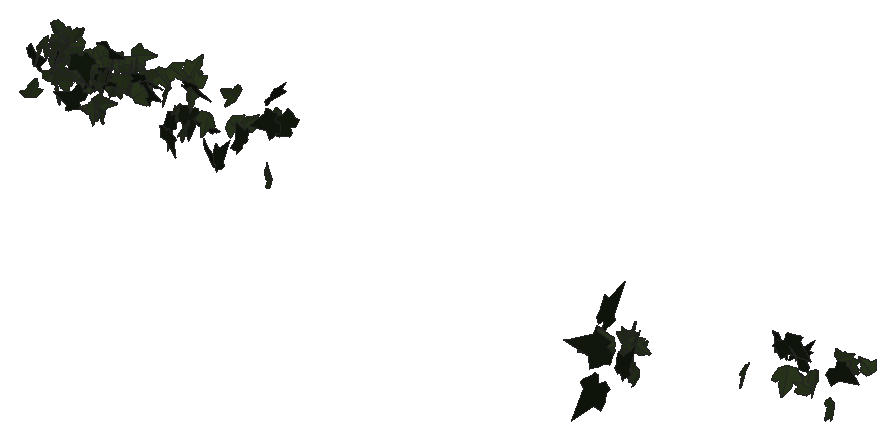
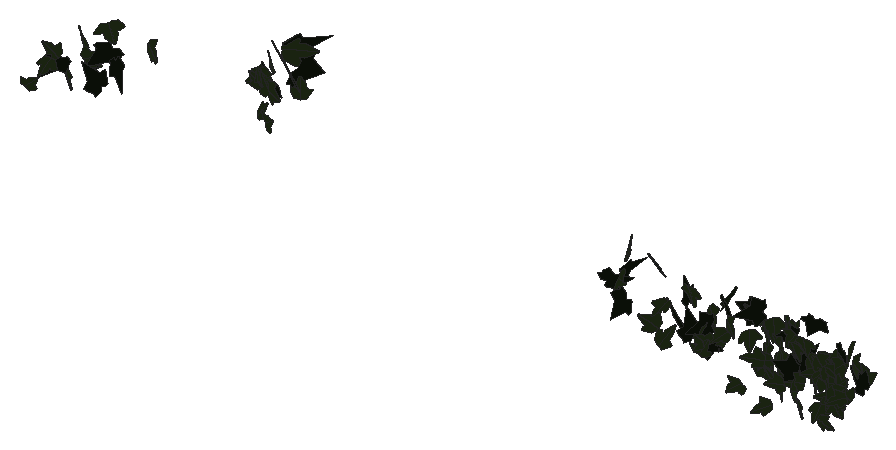
# SketchUp Ruby script. Lengths in inches.
U = 1.inch
M = Sketchup.active_model
def pt(a) = Geom::Point3d.new(a.map { |v| v * U })
def face(e, loops, mat)
  f = e.add_face(loops[0].map { |a| pt(a) })
  loops[1..].each { |l| e.add_face(l.map { |a| pt(a) }).erase! }
  f.material = f.back_material = mat if mat
  f
end
# faces: each face lists its corners as indices into pts; further lists are holes
def faces(e, pts, list, mat = nil) = list.each { |f| face(e, (f[0].is_a?(Array) ? f : [f]).map { |l| l.map { |i| pts[i] } }, mat) }
# xy, xz, yz: faces in a plane at the given z, y or x. An outline is a flat list of corners, or four numbers for a rectangle; further outlines are holes
def ring(l) = l.size == 4 ? [[l[0], l[1]], [l[2], l[1]], [l[2], l[3]], [l[0], l[3]]] : l.each_slice(2).to_a
def flat(e, list, mat, &to3) = list.each { |f| face(e, (f[0].is_a?(Array) ? f : [f]).map { |l| ring(l).map { |u, v| to3.(u, v) } }, mat) }
def xy(e, z, list, mat = nil) = flat(e, list, mat) { |x, y| [x, y, z] }
def xz(e, y, list, mat = nil) = flat(e, list, mat) { |x, z| [x, y, z] }
def yz(e, x, list, mat = nil) = flat(e, list, mat) { |y, z| [x, y, z] }
def lines(e, pts, list) = list.each { |a, b| e.add_line(pt(pts[a]), pt(pts[b])) }
# prism: a flat outline (further loops are holes) pulled along v
def prism(e, loops, v, mat = nil)
  f = face(e, loops, mat); d = Geom::Vector3d.new(v.map { |x| x * U })
  f.pushpull(f.normal.samedirection?(d) ? d.length : -d.length)
end
def box(e, o, s, mat = nil) = prism(e, [[o, [o[0] + s[0], o[1], o[2]], [o[0] + s[0], o[1] + s[1], o[2]], [o[0], o[1] + s[1], o[2]]]], [0, 0, s[2]], mat)
def at(x, y, z, deg = 0) = Geom::Transformation.translation(pt([x, y, z])) * Geom::Transformation.rotation(ORIGIN, Z_AXIS, deg.degrees)
def axes(o, x, y, z) = Geom::Transformation.new([*x, 0, *y, 0, *z, 0, *pt(o).to_a, 1])
def part(name) = M.definitions.add(name)
# library, detail: a bought-in or finely detailed component or shape, given as its bounding box
def library(name, o, s) = part(name).tap { |d| box(d.entities, o, s) }
def detail(e, o, s) = box(e.add_group.entities, o, s)
def put(e, d, t, mat = nil) = e.add_instance(d, t).tap { |i| i.material = mat if mat }
def group(e, t, mat = nil) = e.add_group.tap { |g| g.transformation = t; g.material = mat if mat }.entities
root = M.entities
M.materials.add("efeu1").color = [18, 25, 13]
M.materials.add("efeu2").color = [43, 57, 29]
c1 = part("ivyleaf_10")
p = [[0,0.5,-0.03],[-0.0625,2.02,-0.43],[-0.19,2.01,-0.46],[-0.54,1.05,-0.29],[-0.52,0.625,-0.18],[-0.83,0.76,-0.28],
  [-1.16,0.64,-0.33],[-1.15,0.33,-0.24],[-0.77,-0.39,0.02],[-0.3,-0.51,0.16],[0.04,-0.48,0.23],[-0.02,2.01,-0.4375],
  [-0.06,2.01,-0.43],[0.04,-0.49,0.23],[0.67,-0.49,0.14],[1.38,0.36,-0.2],[1.375,0.51,-0.24],[0.81,0.65,-0.19],
  [0.62,0.59,-0.15],[0.6,1.09,-0.28],[0.5,1.23,-0.31]]
faces(c1.entities,p,[[0,1,2,3,4,5,6,7,8,9,10],[11,12,0,13,14,15,16,17,18,19,20]],"efeu2")
c2 = part("ivyleaf_9")
p = [[1.54,2.16,1.25],[1.36,2.04,1.19],[-0.21,0.99,0.68],[-0.71,1.11,0.82],[-0.85,0.86,0.67],[-0.8,0.17,0.21],
  [-0.9,-0.01,0.1],[-0.67,-0.16,-0.02],[-0.08,-0.08,-0.05],[-0.03,-0.6,-0.4],[0.65,-0.88,-0.66],[0.83,-0.6,-0.49],
  [1.29,-0.42,-0.43],[1.8125,-0.07,-0.26],[1.21,0.44,0.15]]
faces(c2.entities,p,[[0,1,2,3,4,5,6,7,8,9,10,11,12,13,14]],"efeu1")
put(root,c1,axes([519.28,138.82,150.8125],[0.15323,0.09847,0.63212],[0.38291,0.50659,-0.17174],[-0.51249,0.40794,0.06068]))
put(root,c1,axes([519.85,138.97,149.92],[0.47339,0.37363,-0.23743],[-0.18464,-0.14928,-0.60307],[-0.40234,0.50812,-0.00259]))
put(root,c2,axes([519.46,135.91,150.5],[0.0764,-0.09138,0.78277],[0.4972,-0.60459,-0.11911],[0.61145,0.50304,-0.00095]))
put(root,c1,axes([520.43,139.92,148.9],[0.20455,-0.06424,-0.6006],[-0.57771,0.16432,-0.21433],[0.17635,0.61283,-0.00548]))
put(root,c1,axes([520.34,138.58,151.12],[-0.29048,-0.52947,0.26685],[-0.12391,-0.23638,-0.6039],[0.57982,-0.31577,0.00463]))
put(root,c1,axes([520.6,136.84,150.53],[-0.11991,0.37286,0.53038],[-0.20002,0.49179,-0.39096],[-0.6167,-0.232,0.02367]))
put(root,c1,axes([520.39,135.74,152.08],[0.31226,-0.53217,0.51218],[0.25786,-0.44253,-0.61701],[0.69212,0.40496,-0.0012]))
put(root,c1,axes([520.28,137.75,153.01],[-0.52251,0.1784,-0.50215],[0.47077,-0.17499,-0.55204],[-0.2497,-0.70324,0.00998]))
put(root,c1,axes([520.93,137.53,151.31],[-0.24196,-0.66163,0.09856],[-0.03519,-0.09208,-0.70448],[0.66801,-0.2445,-0.00141]))
put(root,c1,axes([520.78,136.25,149.17],[-0.26522,-0.44928,0.37864],[0.18614,0.32978,0.52169],[-0.55729,0.32397,-0.00596]))
put(root,c1,axes([521.37,138.68,149.34],[-0.16271,0.16443,-0.63572],[-0.4383,0.4605,0.23129],[0.48895,0.46751,-0.00423]))
put(root,c1,axes([520.69,137.91,150.44],[0.27064,-0.32237,0.5824],[0.40891,-0.41558,-0.42005],[0.52526,0.48963,0.02692]))
put(root,c1,axes([521.08,139.42,149.67],[-0.46445,-0.38016,-0.22724],[0.1756,0.14424,-0.6002],[0.4066,-0.49653,-0.00037]))
put(root,c1,axes([521.21,137.8,151.26],[0.05305,-0.69928,-0.18249],[-0.01026,0.18224,-0.70128],[0.72263,0.05392,0.00344]))
put(root,c1,axes([521.31,138.21,152.42],[-0.21036,-0.48272,0.36837],[-0.12313,-0.34784,-0.52613],[0.5946,-0.24281,0.02137]))
put(root,c1,axes([521.47,136.4,149.61],[0.43935,-0.46341,-0.33146],[-0.23385,0.23501,-0.63854],[0.51955,0.49766,-0.00712]))
put(root,c1,axes([520.83,138.28,152.01],[0.12747,-0.08265,-0.6202],[0.60457,-0.14678,0.14381],[-0.16118,-0.61592,0.04895]))
put(root,c1,axes([521.54,134.72,152.92],[-0.35621,0.53889,0.4395],[-0.2419,0.36694,-0.64598],[-0.65196,-0.43058,-0.00045]))
put(root,c1,axes([521.27,136.45,151.65],[-0.57958,0.12039,0.3449],[0.3385,-0.06626,0.59194],[0.13738,0.67118,-0.00343]))
put(root,c1,axes([521.39,133.22,149.22],[-0.38018,-0.60564,0.09897],[0.05569,0.08189,0.71507],[-0.61114,0.38422,0.0036]))
put(root,c1,axes([522,137.86,151.08],[-0.11217,-0.53913,0.45324],[-0.12197,-0.43715,-0.55018],[0.6937,-0.16404,-0.02345]))
put(root,c1,axes([522.21,138.11,152.95],[-0.07747,-0.65397,0.2853],[-0.05103,-0.28116,-0.65834],[0.71167,-0.09135,-0.01615]))
put(root,c1,axes([522.25,138.33,151.43],[-0.01249,0.25001,0.63304],[0.03478,-0.63209,0.25032],[0.67973,0.03694,-0.00118]))
put(root,c1,axes([521.82,137.05,149.24],[0.03179,-0.06086,0.66522],[0.52325,0.41626,0.01307],[-0.41525,0.51986,0.06741]))
put(root,c2,axes([522.76,134.5,151.98],[-0.29334,0.20895,-0.70547],[-0.61317,0.35034,0.35873],[0.40666,0.67897,0.032]))
put(root,c1,axes([522.72,134.96,148.48],[-0.16462,0.31635,-0.57425],[-0.27755,0.50277,0.35654],[0.59397,0.32262,0.00745]))
put(root,c1,axes([523.15,134.54,151.41],[-0.08346,-0.55043,-0.56858],[0.12144,0.55605,-0.55613],[0.78199,-0.1451,0.02568]))
put(root,c1,axes([523.82,135.9,151.52],[0.10232,0.00181,-0.71091],[-0.66095,0.26474,-0.09446],[0.2618,0.66766,0.03938]))
put(root,c1,axes([523.25,136.72,150.7],[-0.06403,-0.11847,0.71745],[0.3516,0.62539,0.13465],[-0.63651,0.35737,0.0022]))
put(root,c1,axes([523.77,138.77,148.93],[0.48635,-0.44559,-0.15978],[-0.11213,0.11412,-0.65956],[0.4599,0.49904,0.00816]))
put(root,c1,axes([523.25,134.55,150.44],[-0.3655,-0.1091,0.69788],[0.69173,0.10379,0.37851],[-0.143,0.78093,0.04719]))
put(root,c1,axes([524.48,135.93,149.6],[0.34307,-0.54592,-0.33052],[-0.18009,0.27718,-0.64476],[0.61224,0.38744,-0.00444]))
put(root,c2,axes([524.76,134.91,149],[-0.0473,-0.01374,0.76617],[-0.71265,-0.28136,-0.04904],[0.28166,-0.7142,0.00458]))
put(root,c1,axes([524.8,135.92,151.05],[0.08578,-0.7222,0.17778],[0.01533,-0.1772,-0.72725],[0.7436,0.08696,-0.00551]))
put(root,c1,axes([524.49,138.49,149.54],[0.23113,-0.26019,0.60981],[0.38881,-0.4699,-0.34786],[0.53702,0.45219,-0.0106]))
put(root,c2,axes([524.25,138.86,151.52],[0.31958,-0.15421,0.67829],[0.58557,-0.34327,-0.35394],[0.37546,0.66662,-0.02534]))
put(root,c1,axes([525.07,136.21,152.76],[0.69435,0.04049,0.03455],[0.0345,0.0019,-0.69553],[-0.04054,0.6952,-0.00011]))
put(root,c1,axes([524.78,135.41,150.41],[0.42243,-0.04589,-0.61922],[0.62048,0.00287,0.42308],[-0.02349,-0.74959,0.03953]))
put(root,c2,axes([525.51,136.22,150.41],[0.14984,0.1017,0.75128],[-0.61338,-0.43382,0.18106],[0.44557,-0.63141,-0.00339]))
put(root,c1,axes([525.39,137.1875,152.69],[0.66964,-0.14152,-0.14354],[-0.14068,0.02853,-0.68443],[0.14436,0.68426,-0.00115]))
put(root,c1,axes([524.82,139.68,150.57],[0.15558,0.07308,0.70938],[0.66733,0.2411,-0.17119],[-0.25146,0.68505,-0.01543]))
put(root,c1,axes([525.99,138.32,149.67],[0.30028,-0.55214,-0.34084],[-0.16407,0.29875,-0.62851],[0.62779,0.34218,-0.00123]))
put(root,c1,axes([525.84,135.34,151.9],[-0.32458,-0.31187,-0.51603],[0.38467,0.34418,-0.44997],[0.46431,-0.50317,0.01205]))
put(root,c2,axes([525.76,134.1,153.55],[-0.36013,-0.38511,-0.59413],[0.4411,0.39938,-0.52625],[0.55384,-0.5685,0.03278]))
put(root,c1,axes([525.85,140.02,148.4],[0.12134,0.12235,0.65875],[0.2887,0.59458,-0.16361],[-0.60462,0.30846,0.05408]))
put(root,c1,axes([525.77,139.21,150.63],[0.13979,-0.09929,-0.65288],[0.56403,-0.32916,0.17083],[-0.34349,-0.5809,0.0148]))
put(root,c1,axes([525.87,135.9375,148.68],[0.01511,-0.0893,0.72977],[0.46504,0.56652,0.05969],[-0.56945,0.46027,0.06811]))
put(root,c1,axes([526.26,136.93,150.2],[-0.02624,0.29922,0.63077],[-0.01742,0.63073,-0.29993],[-0.69792,-0.02699,-0.01623]))
put(root,c1,axes([526.56,135.83,148.89],[0.0242,0.02446,-0.67286],[-0.3282,-0.58746,-0.03316],[-0.58789,0.32897,-0.00919]))
put(root,c1,axes([527.09,134.13,149.08],[-0.00863,0.02124,0.74142],[-0.72904,-0.13679,-0.00457],[0.1366,-0.72875,0.02247]))
put(root,c1,axes([526.09,135.29,151.45],[0.00567,0.00174,-0.68587],[0.57809,-0.36912,0.00385],[-0.36909,-0.5781,-0.00452]))
put(root,c1,axes([526.45,135.86,152.6],[0.62395,0.13375,0.4526],[0.44342,0.09078,-0.63811],[-0.16161,0.76545,-0.00341]))
put(root,c1,axes([527.62,136.16,150.59],[-0.51443,0.03771,0.49433],[-0.49479,0.00559,-0.51534],[-0.03106,-0.71342,0.02209]))
put(root,c1,axes([527.4,136.375,150.7],[0.06144,-0.60006,-0.46953],[-0.06153,0.46561,-0.6031],[0.75943,0.08627,-0.01088]))
put(root,c1,axes([526.92,138.55,151.48],[-0.10123,-0.04001,-0.67305],[0.67346,0.02672,-0.10288],[0.03241,-0.6801,0.03555]))
put(root,c1,axes([527.71,133.9,152.02],[-0.15439,0.152,0.68158],[-0.44258,0.51865,-0.21592],[-0.54017,-0.46839,-0.0179]))
put(root,c1,axes([527.57,134.92,152.71],[0.28299,-0.73749,-0.12828],[-0.04111,0.12162,-0.7899],[0.74743,0.28591,0.00512]))
put(root,c1,axes([527.03,139.5,151.91],[-0.08148,-0.04365,0.74271],[0.56265,0.48522,0.09024],[-0.48677,0.56817,-0.02]))
put(root,c1,axes([527.7,137.99,149.67],[0.54286,0.39171,0.27104],[-0.22529,-0.15094,0.66937],[0.41969,-0.58769,0.00873]))
put(root,c2,axes([526.95,134.99,152.09],[0.19712,0.03102,-0.74405],[0.59548,0.45561,0.17676],[0.44718,-0.62039,0.0926]))
put(root,c1,axes([527.23,133.67,150.02],[0.57991,-0.24788,0.42428],[0.39044,-0.16605,-0.63066],[0.29836,0.6991,0.00064]))
put(root,c1,axes([527.8,138.32,151.58],[0.10849,-0.37254,-0.59541],[-0.1209,0.58357,-0.38716],[0.69187,0.16039,0.0257]))
put(root,c1,axes([528.13,134.73,152.9375],[0.25513,-0.60969,-0.39956],[-0.14373,0.37294,-0.66085],[0.71464,0.29267,0.00973]))
put(root,c1,axes([528.18,135.6,151.11],[0.55412,-0.1744,0.3643],[-0.3468,0.11159,0.58091],[-0.20704,-0.65369,0.00197]))
put(root,c1,axes([527.8125,133.83,149.43],[-0.39522,0.09706,0.58681],[0.55217,-0.20199,0.4053],[0.22107,0.67804,0.03674]))
put(root,c1,axes([528.46,136.875,151.34],[0.19846,-0.71041,-0.10598],[-0.0173,0.10519,-0.73752],[0.71806,0.19888,0.01153]))
put(root,c1,axes([528.01,140.9,149.91],[0.42299,0.17543,0.57575],[0.53208,0.21996,-0.45792],[-0.28135,0.67972,-0.00041]))
put(root,c1,axes([528.93,136.14,151.74],[0.50196,-0.45893,0.37581],[-0.27847,0.25238,0.68013],[-0.52375,-0.57402,-0.00143]))
put(root,c1,axes([529.17,135.125,152.54],[-0.56595,-0.51041,0.04357],[-0.03167,-0.02994,-0.76211],[0.51129,-0.56683,0.00102]))
put(root,c1,axes([529.85,137.32,152.22],[-0.47161,-0.55993,0.02203],[-0.00338,-0.02595,-0.73194],[0.56035,-0.47141,0.01412]))
put(root,c2,axes([530.58,134.92,152.96],[0.61995,-0.01156,0.4639],[0.464,0.00372,-0.61998],[0.00702,0.77429,0.00991]))
put(root,c1,axes([531.07,134.43,151.96],[0.47579,0.00884,-0.63596],[0.63585,0.01184,0.47587],[0.01478,-0.79415,0.00002]))
put(root,c1,axes([531.23,138.71,152.42],[0.31623,0.28971,0.5744],[0.38094,0.43144,-0.42733],[-0.51841,0.49375,0.03637]))
put(root,c2,axes([531.49,134.72,152.5],[0.39737,-0.07569,-0.68942],[0.67536,0.22307,0.36477],[0.15786,-0.76383,0.17485]))
put(root,c1,axes([532.08,140.05,151.94],[0.30368,0.44876,-0.52822],[0.25876,0.46159,0.54092],[0.64299,-0.3977,0.03178]))
put(root,c1,axes([532.5,140.09,150.95],[0.64187,0.264,0.30917],[-0.28736,-0.11409,0.69403],[0.28758,-0.70325,0.00347]))
put(root,c1,axes([532.41,136.63,152.01],[0.31407,-0.64295,0.2168],[0.10808,-0.18844,-0.71542],[0.66985,0.33187,0.01379]))
put(root,c1,axes([533.39,136.11,149.96],[0.11314,-0.24235,0.70677],[-0.35097,0.61382,0.26666],[-0.65961,-0.36817,-0.02066]))
put(root,c2,axes([533.36,137.88,152.06],[0.6978,-0.08585,0.31372],[0.30974,-0.05121,-0.70296],[0.09925,0.76336,-0.01187]))
put(root,c1,axes([533.87,137.74,151.73],[-0.04627,0.70809,-0.26757],[0.01701,-0.26702,-0.7096],[-0.75677,-0.0493,0.00041]))
put(root,c2,axes([533.93,137.5,150.0625],[-0.45402,-0.49592,-0.38339],[0.26365,0.2784,-0.67234],[0.56869,-0.52499,0.00562]))
put(root,c2,axes([535.125,133.6875,151.57],[-0.54015,0.06198,-0.66742],[0.66553,-0.05239,-0.54348],[-0.07975,-0.85701,-0.01504]))
put(root,c1,axes([535.97,140.65,150.93],[-0.22632,-0.39702,-0.64952],[-0.32556,-0.56204,0.45699],[-0.68812,0.39649,-0.00258]))
put(root,c1,axes([536.05,134.3,150.88],[0.13656,-0.72766,-0.02306],[-0.00475,0.02257,-0.74036],[0.72801,0.13664,-0.0005]))
put(root,c2,axes([535.78,132.3,151.21],[0.36248,-0.66754,0.13765],[0.06189,-0.12302,-0.75959],[0.67877,0.3677,-0.00425]))
put(root,c2,axes([536,136.76,149.85],[0.77113,0.02402,-0.01539],[0.01467,0.02324,0.77117],[0.02447,-0.77093,0.02277]))
put(root,c1,axes([537.9375,134.6,152.25],[0.80025,-0.1316,-0.0261],[-0.02516,0.00785,-0.81099],[0.13178,0.80064,0.00366]))
put(root,c1,axes([538.76,138.125,150.25],[-0.31512,-0.40181,0.57351],[0.35372,0.45143,0.51064],[-0.60435,0.47373,-0.00017]))
put(root,c2,axes([539.05,134.49,148.66],[-0.32282,0.52243,0.57369],[0.30287,-0.48723,0.61412],[0.71437,0.44266,-0.00112]))
put(root,c1,axes([539.12,136.36,151.34],[0.13615,0.58065,0.5233],[0.12879,0.50725,-0.59636],[-0.77098,0.18727,-0.0072]))
put(root,c2,axes([539.38,133.04,150.14],[-0.04107,-0.1153,0.76827],[0.32378,-0.70188,-0.08803],[0.70618,0.3151,0.08504]))
put(root,c2,axes([540.34,139.76,152.79],[0.21183,0.63216,0.47257],[0.15467,0.44656,-0.6667],[-0.77397,0.26226,-0.0039]))
put(root,c2,axes([542.72,133.11,152.38],[-0.61787,0.1312,-0.46593],[-0.45482,0.1012,0.63164],[0.16565,0.76721,-0.00364]))
put(root,c1,axes([542.59,137.66,152.92],[-0.01233,0.55524,-0.56896],[-0.0118,-0.56909,-0.55511],[-0.79489,-0.00016,0.01707]))
put(root,c2,axes([543.18,136.53,152.92],[0.08196,-0.58274,-0.5782],[0.13303,-0.56396,0.58725],[-0.81006,-0.15157,0.03793]))
put(root,c2,axes([543.96,137.48,152.24],[-0.24417,0.06187,0.76441],[-0.75666,0.11133,-0.2507],[-0.12501,-0.7947,0.02439]))
put(root,c1,axes([546.54,131.72,151.07],[-0.42344,0.50367,0.49473],[0.31753,-0.37938,0.65802],[0.63057,0.52927,0.00087]))
put(root,c2,axes([583.1,128.27,152.75],[-0.53442,0.93859,0.62702],[0.3016,-0.54979,1.08004],[1.08773,0.61359,0.0086]))
put(root,c1,axes([583.41,126.77,150.45],[-0.5932,-0.39198,0.00534],[0.00722,-0.00123,0.71099],[-0.39195,0.59322,0.00501]))
put(root,c1,axes([584.9375,128.78,151.24],[0.1063,-0.08162,-0.8544],[-0.68422,0.5117,-0.13401],[0.51816,0.69243,-0.00168]))
put(root,c1,axes([585.21,128.87,148.24],[0.40863,-0.10104,0.64373],[-0.62413,0.15768,0.42094],[-0.18726,-0.746,0.00178]))
put(root,c1,axes([585.15,128.78,151.22],[0.27287,-0.73795,0.17223],[-0.05993,0.16147,0.78678],[-0.75541,-0.27937,-0.00021]))
put(root,c1,axes([585.97,124.9375,152.7],[-0.10304,0.02593,1.11193],[-0.62614,-0.92428,-0.03647],[0.91924,-0.62666,0.0998]))
put(root,c2,axes([586.03,124.59,152.85],[-0.32069,-0.82047,-0.73409],[-0.21101,-0.70462,0.87971],[-1.08053,0.38111,0.04608]))
put(root,c1,axes([586.11,128.29,152.12],[-0.62787,-0.03152,0.41044],[-0.40852,-0.04428,-0.62835],[0.05059,-0.74881,0.01988]))
put(root,c1,axes([586.3,128.375,152.22],[0.19234,-0.63354,-0.04721],[-0.01422,0.04501,-0.6621],[0.63514,0.19287,-0.00053]))
put(root,c1,axes([585.96,127.13,152.02],[0.39041,-0.44974,-0.38808],[0.2525,-0.29472,0.59555],[-0.5377,-0.46494,-0.00211]))
put(root,c1,axes([586.12,128.49,148.56],[-0.0548,0.11318,0.64234],[0.28304,-0.57662,0.12575],[0.58762,0.28829,-0.00067]))
put(root,c1,axes([586.17,127.51,150.24],[-0.70566,0.16377,0.33641],[0.32784,-0.07548,0.72441],[0.18033,0.77809,-0.00053]))
put(root,c2,axes([586.16,126.59,149.85],[-0.41838,0.52233,0.58323],[0.33752,-0.47635,0.66873],[0.70645,0.53692,0.02591]))
put(root,c2,axes([586.39,123.15,150.14],[0.05363,-0.05264,-1.23871],[0.5891,-1.08989,0.07183],[-1.09093,-0.59113,-0.02211]))
put(root,c1,axes([586.25,128.34,151.1],[-0.41486,-0.25269,0.43967],[0.38714,0.20908,0.48546],[-0.32754,0.56718,0.01692]))
put(root,c1,axes([586.125,128.03,151.72],[-0.39274,-0.09632,-0.65994],[0.65551,0.08539,-0.40257],[0.12291,-0.7632,0.03825]))
put(root,c2,axes([595.7,134.6,152.375],[0.31082,0.09051,-0.77293],[-0.76675,-0.10668,-0.32083],[-0.13305,0.82622,0.04324]))
put(root,c1,axes([595.71,130.26,151.86],[0.29374,-0.69674,0.27974],[0.12623,-0.25029,-0.75591],[0.74011,0.31922,0.0179]))
put(root,c2,axes([596.42,135.78,150.71],[0.41557,0.67091,0.04072],[-0.02505,-0.03238,0.78918],[0.67168,-0.41631,0.00423]))
put(root,c2,axes([596.73,134.05,152.97],[-0.04672,-0.17198,-0.85274],[0.33287,0.78544,-0.17665],[0.8037,-0.3353,0.02359]))
put(root,c2,axes([597.57,135.37,150.96],[0.15283,-0.7994,0.07284],[0.00137,0.07441,0.81373],[-0.80271,-0.15207,0.01526]))
put(root,c1,axes([599.9,132.79,150.53],[0.34085,0.34409,0.74858],[-0.6325,-0.40983,0.47637],[0.52793,-0.71316,0.08743]))
put(root,c1,axes([599.56,130.63,152.65],[0.65837,0.68502,-0.18949],[-0.13076,-0.13715,-0.95011],[-0.69862,0.67123,-0.00075]))
put(root,c2,axes([600.78,135.36,151.3125],[0.0347,-0.19447,-0.75689],[0.05806,0.75618,-0.19163],[0.77932,-0.04768,0.04798]))
put(root,c1,axes([600.93,132.36,152.1],[0.66,-0.412,0.30493],[0.25105,-0.17358,-0.77792],[0.44687,0.70601,-0.01332]))
put(root,c1,axes([600.79,135.91,152],[-0.38277,-0.1538,0.55478],[0.51301,0.2112,0.4125],[-0.26125,0.64007,-0.00281]))
put(root,c1,axes([601.11,136.42,151.45],[-0.39301,-0.40252,-0.36821],[0.28725,0.23311,-0.56143],[0.46378,-0.48549,0.03571]))
put(root,c1,axes([601.54,138.53,150.12],[0.40593,0.26107,0.41751],[-0.38022,-0.17765,0.48076],[0.3129,-0.55456,0.04254]))
put(root,c1,axes([601.75,133.41,149.14],[0.59308,-0.48205,-0.26083],[-0.18336,0.18766,-0.76374],[0.51651,0.62013,0.02837]))
